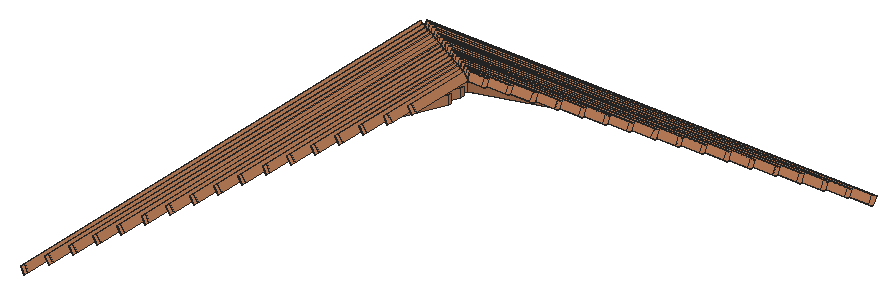
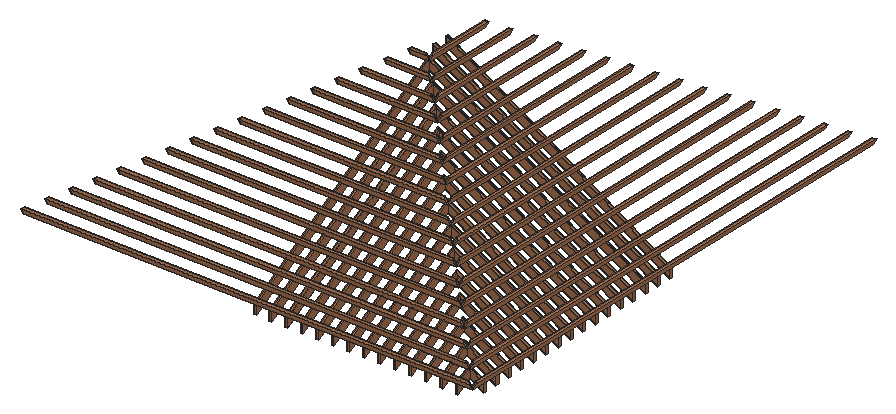
# SketchUp Ruby script. Lengths in millimetres.
U = 1.mm
M = Sketchup.active_model
def pt(a) = Geom::Point3d.new(a.map { |v| v * U })
def face(e, loops, mat)
  f = e.add_face(loops[0].map { |a| pt(a) })
  loops[1..].each { |l| e.add_face(l.map { |a| pt(a) }).erase! }
  f.material = f.back_material = mat if mat
  f
end
# faces: each face lists its corners as indices into pts; further lists are holes
def faces(e, pts, list, mat = nil) = list.each { |f| face(e, (f[0].is_a?(Array) ? f : [f]).map { |l| l.map { |i| pts[i] } }, mat) }
# xy, xz, yz: faces in a plane at the given z, y or x. An outline is a flat list of corners, or four numbers for a rectangle; further outlines are holes
def ring(l) = l.size == 4 ? [[l[0], l[1]], [l[2], l[1]], [l[2], l[3]], [l[0], l[3]]] : l.each_slice(2).to_a
def flat(e, list, mat, &to3) = list.each { |f| face(e, (f[0].is_a?(Array) ? f : [f]).map { |l| ring(l).map { |u, v| to3.(u, v) } }, mat) }
def xy(e, z, list, mat = nil) = flat(e, list, mat) { |x, y| [x, y, z] }
def xz(e, y, list, mat = nil) = flat(e, list, mat) { |x, z| [x, y, z] }
def yz(e, x, list, mat = nil) = flat(e, list, mat) { |y, z| [x, y, z] }
def lines(e, pts, list) = list.each { |a, b| e.add_line(pt(pts[a]), pt(pts[b])) }
# prism: a flat outline (further loops are holes) pulled along v
def prism(e, loops, v, mat = nil)
  f = face(e, loops, mat); d = Geom::Vector3d.new(v.map { |x| x * U })
  f.pushpull(f.normal.samedirection?(d) ? d.length : -d.length)
end
def box(e, o, s, mat = nil) = prism(e, [[o, [o[0] + s[0], o[1], o[2]], [o[0] + s[0], o[1] + s[1], o[2]], [o[0], o[1] + s[1], o[2]]]], [0, 0, s[2]], mat)
def at(x, y, z, deg = 0) = Geom::Transformation.translation(pt([x, y, z])) * Geom::Transformation.rotation(ORIGIN, Z_AXIS, deg.degrees)
def axes(o, x, y, z) = Geom::Transformation.new([*x, 0, *y, 0, *z, 0, *pt(o).to_a, 1])
def part(name) = M.definitions.add(name)
# library, detail: a bought-in or finely detailed component or shape, given as its bounding box
def library(name, o, s) = part(name).tap { |d| box(d.entities, o, s) }
def detail(e, o, s) = box(e.add_group.entities, o, s)
def put(e, d, t, mat = nil) = e.add_instance(d, t).tap { |i| i.material = mat if mat }
def group(e, t, mat = nil) = e.add_group.tap { |g| g.transformation = t; g.material = mat if mat }.entities
root = M.entities
M.materials.add("[Wood Veneer 02]").color = [190, 128, 91]
c1 = part("Group162\#1")
xy(c1.entities,0,[[-322.7,-9540.5,-381.6,-9489.5,0,-9489.5,0,-9540.5]])
xy(c1.entities,152,[[-410.5,-9540.5,-87.8,-9540.5,-87.8,-9489.5,-469.4,-9489.5]])
xz(c1.entities,-9540.5,[[-322.7,0,0,0,-87.8,152,-410.5,152]])
xz(c1.entities,-9489.5,[[-381.6,0,-469.4,152,-87.8,152,0,0]])
p = [[-381.6,-9489.5,0],[-322.7,-9540.5,0],[-410.5,-9540.5,152],[-469.4,-9489.5,152],[0,-9540.5,0],[0,-9489.5,0],
  [-87.8,-9489.5,152],[-87.8,-9540.5,152]]
faces(c1.entities,p,[[0,1,2,3],[4,5,6,7]])
c2 = part("Group115\#1")
xy(c2.entities,0,[[-381.6,-330.5,-322.7,-279.5,0,-279.5,0,-330.5]])
xy(c2.entities,152,[[-469.4,-330.5,-87.8,-330.5,-87.8,-279.5,-410.5,-279.5]])
xz(c2.entities,-330.5,[[-381.6,0,0,0,-87.8,152,-469.4,152]])
xz(c2.entities,-279.5,[[-322.7,0,-410.5,152,-87.8,152,0,0]])
p = [[-381.6,-330.5,0],[-469.4,-330.5,152],[-410.5,-279.5,152],[-322.7,-279.5,0],[-87.8,-330.5,152],[0,-330.5,0],
  [0,-279.5,0],[-87.8,-279.5,152]]
faces(c2.entities,p,[[0,1,2,3],[4,5,6,7]])
c3 = part("Group164\#1")
xy(c3.entities,0,[[-674.9,-9235.5,-733.8,-9184.5,0,-9184.5,0,-9235.5]])
xy(c3.entities,152,[[-762.7,-9235.5,-87.8,-9235.5,-87.8,-9184.5,-821.6,-9184.5]])
xz(c3.entities,-9235.5,[[-674.9,0,0,0,-87.8,152,-762.7,152]])
xz(c3.entities,-9184.5,[[-733.8,0,-821.6,152,-87.8,152,0,0]])
p = [[-674.9,-9235.5,0],[-762.7,-9235.5,152],[-821.6,-9184.5,152],[-733.8,-9184.5,0],[-87.8,-9235.5,152],[0,-9235.5,0],
  [0,-9184.5,0],[-87.8,-9184.5,152]]
faces(c3.entities,p,[[0,1,2,3],[4,5,6,7]])
c4 = part("Group166\#1")
xy(c4.entities,0,[[-1027.1,-8930.5,-1086,-8879.5,0,-8879.5,0,-8930.5]])
xy(c4.entities,152,[[-1114.9,-8930.5,-87.8,-8930.5,-87.8,-8879.5,-1173.8,-8879.5]])
xz(c4.entities,-8930.5,[[-1027.1,0,0,0,-87.8,152,-1114.9,152]])
xz(c4.entities,-8879.5,[[-1086,0,-1173.8,152,-87.8,152,0,0]])
p = [[-1086,-8879.5,0],[-1027.1,-8930.5,0],[-1114.9,-8930.5,152],[-1173.8,-8879.5,152],[0,-8930.5,0],[0,-8879.5,0],
  [-87.8,-8879.5,152],[-87.8,-8930.5,152]]
faces(c4.entities,p,[[0,1,2,3],[4,5,6,7]])
c5 = part("Group117\#1")
xy(c5.entities,0,[[-733.8,-635.5,-674.9,-584.5,0,-584.5,0,-635.5]])
xy(c5.entities,152,[[-821.6,-635.5,-87.8,-635.5,-87.8,-584.5,-762.7,-584.5]])
xz(c5.entities,-635.5,[[-733.8,0,0,0,-87.8,152,-821.6,152]])
xz(c5.entities,-584.5,[[-674.9,0,-762.7,152,-87.8,152,0,0]])
p = [[-762.7,-584.5,152],[-674.9,-584.5,0],[-733.8,-635.5,0],[-821.6,-635.5,152],[0,-584.5,0],[-87.8,-584.5,152],
  [-87.8,-635.5,152],[0,-635.5,0]]
faces(c5.entities,p,[[0,1,2,3],[4,5,6,7]])
c6 = part("Group168\#1")
xy(c6.entities,0,[[-1379.3,-8625.5,-1438.2,-8574.5,0,-8574.5,0,-8625.5]])
xy(c6.entities,152,[[-1467,-8625.5,-87.8,-8625.5,-87.8,-8574.5,-1525.9,-8574.5]])
xz(c6.entities,-8625.5,[[-1379.3,0,0,0,-87.8,152,-1467,152]])
xz(c6.entities,-8574.5,[[-1438.2,0,-1525.9,152,-87.8,152,0,0]])
p = [[-1379.3,-8625.5,0],[-1467,-8625.5,152],[-1525.9,-8574.5,152],[-1438.2,-8574.5,0],[-87.8,-8625.5,152],[0,-8625.5,0],
  [0,-8574.5,0],[-87.8,-8574.5,152]]
faces(c6.entities,p,[[0,1,2,3],[4,5,6,7]])
c7 = part("Group170\#1")
xy(c7.entities,0,[[-1731.5,-8320.5,-1790.4,-8269.5,0,-8269.5,0,-8320.5]])
xy(c7.entities,152,[[-1819.2,-8320.5,-87.8,-8320.5,-87.8,-8269.5,-1878.1,-8269.5]])
xz(c7.entities,-8320.5,[[-1731.5,0,0,0,-87.8,152,-1819.2,152]])
xz(c7.entities,-8269.5,[[-1790.4,0,-1878.1,152,-87.8,152,0,0]])
p = [[-1819.2,-8320.5,152],[-1878.1,-8269.5,152],[-1790.4,-8269.5,0],[-1731.5,-8320.5,0],[-87.8,-8269.5,152],[-87.8,-8320.5,152],
  [0,-8320.5,0],[0,-8269.5,0]]
faces(c7.entities,p,[[0,1,2,3],[4,5,6,7]])
c8 = part("Group119\#1")
xy(c8.entities,0,[[-1086,-940.5,-1027.1,-889.5,0,-889.5,0,-940.5]])
xy(c8.entities,152,[[-1173.8,-940.5,-87.8,-940.5,-87.8,-889.5,-1114.9,-889.5]])
xz(c8.entities,-940.5,[[-1086,0,0,0,-87.8,152,-1173.8,152]])
xz(c8.entities,-889.5,[[-1027.1,0,-1114.9,152,-87.8,152,0,0]])
p = [[-1114.9,-889.5,152],[-1027.1,-889.5,0],[-1086,-940.5,0],[-1173.8,-940.5,152],[0,-889.5,0],[-87.8,-889.5,152],
  [-87.8,-940.5,152],[0,-940.5,0]]
faces(c8.entities,p,[[0,1,2,3],[4,5,6,7]])
c9 = part("Group172\#1")
xy(c9.entities,0,[[-2083.7,-8015.5,-2142.5,-7964.5,0,-7964.5,0,-8015.5]])
xy(c9.entities,152,[[-2171.4,-8015.5,-87.8,-8015.5,-87.8,-7964.5,-2230.3,-7964.5]])
xz(c9.entities,-8015.5,[[-2083.7,0,0,0,-87.8,152,-2171.4,152]])
xz(c9.entities,-7964.5,[[-2142.5,0,-2230.3,152,-87.8,152,0,0]])
p = [[-2171.4,-8015.5,152],[-2230.3,-7964.5,152],[-2142.5,-7964.5,0],[-2083.7,-8015.5,0],[-87.8,-7964.5,152],[-87.8,-8015.5,152],
  [0,-8015.5,0],[0,-7964.5,0]]
faces(c9.entities,p,[[0,1,2,3],[4,5,6,7]])
c10 = part("Group174\#1")
xy(c10.entities,0,[[-2435.8,-7710.5,-2494.7,-7659.5,0,-7659.5,0,-7710.5]])
xy(c10.entities,152,[[-2523.6,-7710.5,-87.8,-7710.5,-87.8,-7659.5,-2582.5,-7659.5]])
xz(c10.entities,-7710.5,[[-2435.8,0,0,0,-87.8,152,-2523.6,152]])
xz(c10.entities,-7659.5,[[-2494.7,0,-2582.5,152,-87.8,152,0,0]])
p = [[-2435.8,-7710.5,0],[-2523.6,-7710.5,152],[-2582.5,-7659.5,152],[-2494.7,-7659.5,0],[-87.8,-7710.5,152],[0,-7710.5,0],
  [0,-7659.5,0],[-87.8,-7659.5,152]]
faces(c10.entities,p,[[0,1,2,3],[4,5,6,7]])
c11 = part("Group121\#1")
xy(c11.entities,0,[[-1438.2,-1245.5,-1379.3,-1194.5,0,-1194.5,0,-1245.5]])
xy(c11.entities,152,[[-1525.9,-1245.5,-87.8,-1245.5,-87.8,-1194.5,-1467,-1194.5]])
xz(c11.entities,-1245.5,[[-1438.2,0,0,0,-87.8,152,-1525.9,152]])
xz(c11.entities,-1194.5,[[-1379.3,0,-1467,152,-87.8,152,0,0]])
p = [[-1379.3,-1194.5,0],[-1438.2,-1245.5,0],[-1525.9,-1245.5,152],[-1467,-1194.5,152],[0,-1245.5,0],[0,-1194.5,0],
  [-87.8,-1194.5,152],[-87.8,-1245.5,152]]
faces(c11.entities,p,[[0,1,2,3],[4,5,6,7]])
c12 = part("Group176\#1")
xy(c12.entities,0,[[-2788,-7405.5,-2846.9,-7354.5,0,-7354.5,0,-7405.5]])
xy(c12.entities,152,[[-2875.8,-7405.5,-87.8,-7405.5,-87.8,-7354.5,-2934.7,-7354.5]])
xz(c12.entities,-7405.5,[[-2788,0,0,0,-87.8,152,-2875.8,152]])
xz(c12.entities,-7354.5,[[-2846.9,0,-2934.7,152,-87.8,152,0,0]])
p = [[-2788,-7405.5,0],[-2875.8,-7405.5,152],[-2934.7,-7354.5,152],[-2846.9,-7354.5,0],[-87.8,-7405.5,152],[0,-7405.5,0],
  [0,-7354.5,0],[-87.8,-7354.5,152]]
faces(c12.entities,p,[[0,1,2,3],[4,5,6,7]])
c13 = part("Group178\#1")
xy(c13.entities,0,[[-3140.2,-7100.5,-3199.1,-7049.5,0,-7049.5,0,-7100.5]])
xy(c13.entities,152,[[-3228,-7100.5,-87.8,-7100.5,-87.8,-7049.5,-3286.9,-7049.5]])
xz(c13.entities,-7100.5,[[-3140.2,0,0,0,-87.8,152,-3228,152]])
xz(c13.entities,-7049.5,[[-3199.1,0,-3286.9,152,-87.8,152,0,0]])
p = [[-3228,-7100.5,152],[-3286.9,-7049.5,152],[-3199.1,-7049.5,0],[-3140.2,-7100.5,0],[-87.8,-7049.5,152],[-87.8,-7100.5,152],
  [0,-7100.5,0],[0,-7049.5,0]]
faces(c13.entities,p,[[0,1,2,3],[4,5,6,7]])
c14 = part("Group123\#1")
xy(c14.entities,0,[[-1790.4,-1550.5,-1731.5,-1499.5,0,-1499.5,0,-1550.5]])
xy(c14.entities,152,[[-1878.1,-1550.5,-87.8,-1550.5,-87.8,-1499.5,-1819.2,-1499.5]])
xz(c14.entities,-1550.5,[[-1790.4,0,0,0,-87.8,152,-1878.1,152]])
xz(c14.entities,-1499.5,[[-1731.5,0,-1819.2,152,-87.8,152,0,0]])
p = [[-1878.1,-1550.5,152],[-1819.2,-1499.5,152],[-1731.5,-1499.5,0],[-1790.4,-1550.5,0],[-87.8,-1499.5,152],[-87.8,-1550.5,152],
  [0,-1550.5,0],[0,-1499.5,0]]
faces(c14.entities,p,[[0,1,2,3],[4,5,6,7]])
c15 = part("Group180\#1")
xy(c15.entities,0,[[-3492.4,-6795.5,-3551.3,-6744.5,0,-6744.5,0,-6795.5]])
xy(c15.entities,152,[[-3580.1,-6795.5,-87.8,-6795.5,-87.8,-6744.5,-3639,-6744.5]])
xz(c15.entities,-6795.5,[[-3492.4,0,0,0,-87.8,152,-3580.1,152]])
xz(c15.entities,-6744.5,[[-3551.3,0,-3639,152,-87.8,152,0,0]])
p = [[-3551.3,-6744.5,0],[-3492.4,-6795.5,0],[-3580.1,-6795.5,152],[-3639,-6744.5,152],[0,-6795.5,0],[0,-6744.5,0],
  [-87.8,-6744.5,152],[-87.8,-6795.5,152]]
faces(c15.entities,p,[[0,1,2,3],[4,5,6,7]])
c16 = part("Group182\#1")
xy(c16.entities,0,[[-3844.6,-6490.5,-3903.5,-6439.5,0,-6439.5,0,-6490.5]])
xy(c16.entities,152,[[-3932.3,-6490.5,-87.8,-6490.5,-87.8,-6439.5,-3991.2,-6439.5]])
xz(c16.entities,-6490.5,[[-3844.6,0,0,0,-87.8,152,-3932.3,152]])
xz(c16.entities,-6439.5,[[-3903.5,0,-3991.2,152,-87.8,152,0,0]])
p = [[-3903.5,-6439.5,0],[-3844.6,-6490.5,0],[-3932.3,-6490.5,152],[-3991.2,-6439.5,152],[0,-6490.5,0],[0,-6439.5,0],
  [-87.8,-6439.5,152],[-87.8,-6490.5,152]]
faces(c16.entities,p,[[0,1,2,3],[4,5,6,7]])
c17 = part("Group125\#1")
xy(c17.entities,0,[[-2142.5,-1855.5,-2083.7,-1804.5,0,-1804.5,0,-1855.5]])
xy(c17.entities,152,[[-2230.3,-1855.5,-87.8,-1855.5,-87.8,-1804.5,-2171.4,-1804.5]])
xz(c17.entities,-1855.5,[[-2142.5,0,0,0,-87.8,152,-2230.3,152]])
xz(c17.entities,-1804.5,[[-2083.7,0,-2171.4,152,-87.8,152,0,0]])
p = [[-2171.4,-1804.5,152],[-2083.7,-1804.5,0],[-2142.5,-1855.5,0],[-2230.3,-1855.5,152],[0,-1804.5,0],[-87.8,-1804.5,152],
  [-87.8,-1855.5,152],[0,-1855.5,0]]
faces(c17.entities,p,[[0,1,2,3],[4,5,6,7]])
c18 = part("Group184\#1")
xy(c18.entities,0,[[-4196.8,-6185.5,-4255.6,-6134.5,0,-6134.5,0,-6185.5]])
xy(c18.entities,152,[[-4284.5,-6185.5,-87.8,-6185.5,-87.8,-6134.5,-4343.4,-6134.5]])
xz(c18.entities,-6185.5,[[-4196.8,0,0,0,-87.8,152,-4284.5,152]])
xz(c18.entities,-6134.5,[[-4255.6,0,-4343.4,152,-87.8,152,0,0]])
p = [[-4343.4,-6134.5,152],[-4255.6,-6134.5,0],[-4196.8,-6185.5,0],[-4284.5,-6185.5,152],[0,-6134.5,0],[-87.8,-6134.5,152],
  [-87.8,-6185.5,152],[0,-6185.5,0]]
faces(c18.entities,p,[[0,1,2,3],[4,5,6,7]])
c19 = part("Group186\#1")
xy(c19.entities,0,[[-4548.9,-5880.5,-4607.8,-5829.5,0,-5829.5,0,-5880.5]])
xy(c19.entities,152,[[-4636.7,-5880.5,-87.8,-5880.5,-87.8,-5829.5,-4695.6,-5829.5]])
xz(c19.entities,-5880.5,[[-4548.9,0,0,0,-87.8,152,-4636.7,152]])
xz(c19.entities,-5829.5,[[-4607.8,0,-4695.6,152,-87.8,152,0,0]])
p = [[-4607.8,-5829.5,0],[-4548.9,-5880.5,0],[-4636.7,-5880.5,152],[-4695.6,-5829.5,152],[0,-5880.5,0],[0,-5829.5,0],
  [-87.8,-5829.5,152],[-87.8,-5880.5,152]]
faces(c19.entities,p,[[0,1,2,3],[4,5,6,7]])
c20 = part("Group195\#1")
prism(c20.entities,[[[-4865.8,-2495.1,0],[4865.8,-2495.1,0],[4910,-2546.1,0],[-4910,-2546.1,0]]],[0,0,152])
c21 = part("Group196\#1")
prism(c21.entities,[[[4645.9,-2241.1,0],[-4645.9,-2241.1,0],[-4601.7,-2190.1,0],[4601.7,-2190.1,0]]],[0,0,152])
c22 = part("Group197\#1")
prism(c22.entities,[[[-4337.6,-1885.1,0],[4337.6,-1885.1,0],[4381.7,-1936.1,0],[-4381.7,-1936.1,0]]],[0,0,152])
c23 = part("Group198\#1")
prism(c23.entities,[[[-4073.4,-1580.1,0],[4073.4,-1580.1,0],[4117.6,-1631.1,0],[-4117.6,-1631.1,0]]],[0,0,152])
c24 = part("Group199\#1")
prism(c24.entities,[[[-3809.3,-1275.1,0],[3809.3,-1275.1,0],[3853.4,-1326.1,0],[-3853.4,-1326.1,0]]],[0,0,152])
c25 = part("Group200\#1")
prism(c25.entities,[[[3589.3,-1021.1,0],[-3589.3,-1021.1,0],[-3545.1,-970.1,0],[3545.1,-970.1,0]]],[0,0,152])
c26 = part("Group201\#1")
prism(c26.entities,[[[3325.2,-716.1,0],[-3325.2,-716.1,0],[-3281,-665.1,0],[3281,-665.1,0]]],[0,0,152])
c27 = part("Group202\#1")
prism(c27.entities,[[[-3016.9,-360.1,0],[3016.9,-360.1,0],[3061,-411.1,0],[-3061,-411.1,0]]],[0,0,152])
c28 = part("Group203\#1")
prism(c28.entities,[[[2796.9,-106.1,0],[-2796.9,-106.1,0],[-2752.7,-55.1,0],[2752.7,-55.1,0]]],[0,0,152])
c29 = part("Group204\#1")
prism(c29.entities,[[[2532.8,198.9,0],[-2532.8,198.9,0],[-2488.6,249.9,0],[2488.6,249.9,0]]],[0,0,152])
c30 = part("Group205\#1")
prism(c30.entities,[[[-2224.5,554.9,0],[2224.5,554.9,0],[2268.6,503.9,0],[-2268.6,503.9,0]]],[0,0,152])
c31 = part("Group206\#1")
prism(c31.entities,[[[-1960.3,859.9,0],[1960.3,859.9,0],[2004.5,808.9,0],[-2004.5,808.9,0]]],[0,0,152])
c32 = part("Group207\#1")
prism(c32.entities,[[[-1696.2,1164.9,0],[1696.2,1164.9,0],[1740.3,1113.9,0],[-1740.3,1113.9,0]]],[0,0,152])
c33 = part("Group208\#1")
prism(c33.entities,[[[-1432,1469.9,0],[1432,1469.9,0],[1476.2,1418.9,0],[-1476.2,1418.9,0]]],[0,0,152])
c34 = part("Group209\#1")
prism(c34.entities,[[[-1167.9,1774.9,0],[1167.9,1774.9,0],[1212.1,1723.9,0],[-1212.1,1723.9,0]]],[0,0,152])
c35 = part("Group210\#1")
prism(c35.entities,[[[-903.8,2079.9,0],[903.8,2079.9,0],[947.9,2028.9,0],[-947.9,2028.9,0]]],[0,0,152])
c36 = part("Group211\#1")
prism(c36.entities,[[[-639.6,2384.9,0],[639.6,2384.9,0],[683.8,2333.9,0],[-683.8,2333.9,0]]],[0,0,152])
c37 = part("Group193\#2")
put(c37.entities,c20,at(0,0,0))
put(c37.entities,c21,at(0,0,0))
put(c37.entities,c22,at(0,0,0))
put(c37.entities,c23,at(0,0,0))
put(c37.entities,c24,at(0,0,0))
put(c37.entities,c25,at(0,0,0))
put(c37.entities,c26,at(0,0,0))
put(c37.entities,c27,at(0,0,0))
put(c37.entities,c28,at(0,0,0))
put(c37.entities,c29,at(0,0,0))
put(c37.entities,c30,at(0,0,0))
put(c37.entities,c31,at(0,0,0))
put(c37.entities,c32,at(0,0,0))
put(c37.entities,c33,at(0,0,0))
put(c37.entities,c34,at(0,0,0))
put(c37.entities,c35,at(0,0,0))
put(c37.entities,c36,at(0,0,0))
c38 = part("Group127\#1")
xy(c38.entities,0,[[-2494.7,-2160.5,-2435.8,-2109.5,0,-2109.5,0,-2160.5]])
xy(c38.entities,152,[[-2582.5,-2160.5,-87.8,-2160.5,-87.8,-2109.5,-2523.6,-2109.5]])
xz(c38.entities,-2160.5,[[-2494.7,0,0,0,-87.8,152,-2582.5,152]])
xz(c38.entities,-2109.5,[[-2435.8,0,-2523.6,152,-87.8,152,0,0]])
p = [[-2435.8,-2109.5,0],[-2494.7,-2160.5,0],[-2582.5,-2160.5,152],[-2523.6,-2109.5,152],[0,-2160.5,0],[0,-2109.5,0],
  [-87.8,-2109.5,152],[-87.8,-2160.5,152]]
faces(c38.entities,p,[[0,1,2,3],[4,5,6,7]])
c39 = part("Group188\#1")
xy(c39.entities,0,[[-4901.1,-5575.5,-4960,-5524.5,0,-5524.5,0,-5575.5]])
xy(c39.entities,152,[[-4988.9,-5575.5,-87.8,-5575.5,-87.8,-5524.5,-5047.8,-5524.5]])
xz(c39.entities,-5575.5,[[-4901.1,0,0,0,-87.8,152,-4988.9,152]])
xz(c39.entities,-5524.5,[[-4960,0,-5047.8,152,-87.8,152,0,0]])
p = [[-4960,-5524.5,0],[-4901.1,-5575.5,0],[-4988.9,-5575.5,152],[-5047.8,-5524.5,152],[0,-5575.5,0],[0,-5524.5,0],
  [-87.8,-5524.5,152],[-87.8,-5575.5,152]]
faces(c39.entities,p,[[0,1,2,3],[4,5,6,7]])
c40 = part("Group192\#1")
prism(c40.entities,[[[-87.8,-4965.5,152],[-5180,-4965.5,152],[-5092.2,-4965.5,0],[0,-4965.5,0]]],[0,51,0])
c41 = part("Group190\#1")
prism(c41.entities,[[[-5180,-5219.5,152],[-87.8,-5219.5,152],[0,-5219.5,0],[-5092.2,-5219.5,0]]],[0,-51,0])
c42 = part("Group129\#1")
xy(c42.entities,0,[[-2846.9,-2465.5,-2788,-2414.5,0,-2414.5,0,-2465.5]])
xy(c42.entities,152,[[-2934.7,-2465.5,-87.8,-2465.5,-87.8,-2414.5,-2875.8,-2414.5]])
xz(c42.entities,-2465.5,[[-2846.9,0,0,0,-87.8,152,-2934.7,152]])
xz(c42.entities,-2414.5,[[-2788,0,-2875.8,152,-87.8,152,0,0]])
p = [[-2934.7,-2465.5,152],[-2875.8,-2414.5,152],[-2788,-2414.5,0],[-2846.9,-2465.5,0],[-87.8,-2414.5,152],[-87.8,-2465.5,152],
  [0,-2465.5,0],[0,-2414.5,0]]
faces(c42.entities,p,[[0,1,2,3],[4,5,6,7]])
c43 = part("Group131\#1")
xy(c43.entities,0,[[-3199.1,-2770.5,-3140.2,-2719.5,0,-2719.5,0,-2770.5]])
xy(c43.entities,152,[[-3286.9,-2770.5,-87.8,-2770.5,-87.8,-2719.5,-3228,-2719.5]])
xz(c43.entities,-2770.5,[[-3199.1,0,0,0,-87.8,152,-3286.9,152]])
xz(c43.entities,-2719.5,[[-3140.2,0,-3228,152,-87.8,152,0,0]])
p = [[-3140.2,-2719.5,0],[-3199.1,-2770.5,0],[-3286.9,-2770.5,152],[-3228,-2719.5,152],[0,-2770.5,0],[0,-2719.5,0],
  [-87.8,-2719.5,152],[-87.8,-2770.5,152]]
faces(c43.entities,p,[[0,1,2,3],[4,5,6,7]])
c44 = part("Group133\#1")
xy(c44.entities,0,[[-3551.3,-3075.5,-3492.4,-3024.5,0,-3024.5,0,-3075.5]])
xy(c44.entities,152,[[-3639,-3075.5,-87.8,-3075.5,-87.8,-3024.5,-3580.1,-3024.5]])
xz(c44.entities,-3075.5,[[-3551.3,0,0,0,-87.8,152,-3639,152]])
xz(c44.entities,-3024.5,[[-3492.4,0,-3580.1,152,-87.8,152,0,0]])
p = [[-3551.3,-3075.5,0],[-3639,-3075.5,152],[-3580.1,-3024.5,152],[-3492.4,-3024.5,0],[-87.8,-3075.5,152],[0,-3075.5,0],
  [0,-3024.5,0],[-87.8,-3024.5,152]]
faces(c44.entities,p,[[0,1,2,3],[4,5,6,7]])
c45 = part("Group135\#1")
xy(c45.entities,0,[[-3903.5,-3380.5,-3844.6,-3329.5,0,-3329.5,0,-3380.5]])
xy(c45.entities,152,[[-3991.2,-3380.5,-87.8,-3380.5,-87.8,-3329.5,-3932.3,-3329.5]])
xz(c45.entities,-3380.5,[[-3903.5,0,0,0,-87.8,152,-3991.2,152]])
xz(c45.entities,-3329.5,[[-3844.6,0,-3932.3,152,-87.8,152,0,0]])
p = [[-3903.5,-3380.5,0],[-3991.2,-3380.5,152],[-3932.3,-3329.5,152],[-3844.6,-3329.5,0],[-87.8,-3380.5,152],[0,-3380.5,0],
  [0,-3329.5,0],[-87.8,-3329.5,152]]
faces(c45.entities,p,[[0,1,2,3],[4,5,6,7]])
c46 = part("Group137\#1")
xy(c46.entities,0,[[-4255.6,-3685.5,-4196.8,-3634.5,0,-3634.5,0,-3685.5]])
xy(c46.entities,152,[[-4343.4,-3685.5,-87.8,-3685.5,-87.8,-3634.5,-4284.5,-3634.5]])
xz(c46.entities,-3685.5,[[-4255.6,0,0,0,-87.8,152,-4343.4,152]])
xz(c46.entities,-3634.5,[[-4196.8,0,-4284.5,152,-87.8,152,0,0]])
p = [[-4343.4,-3685.5,152],[-4284.5,-3634.5,152],[-4196.8,-3634.5,0],[-4255.6,-3685.5,0],[-87.8,-3634.5,152],[-87.8,-3685.5,152],
  [0,-3685.5,0],[0,-3634.5,0]]
faces(c46.entities,p,[[0,1,2,3],[4,5,6,7]])
c47 = part("Group139\#1")
xy(c47.entities,0,[[-4607.8,-3990.5,-4548.9,-3939.5,0,-3939.5,0,-3990.5]])
xy(c47.entities,152,[[-4695.6,-3990.5,-87.8,-3990.5,-87.8,-3939.5,-4636.7,-3939.5]])
xz(c47.entities,-3990.5,[[-4607.8,0,0,0,-87.8,152,-4695.6,152]])
xz(c47.entities,-3939.5,[[-4548.9,0,-4636.7,152,-87.8,152,0,0]])
p = [[-4695.6,-3990.5,152],[-4636.7,-3939.5,152],[-4548.9,-3939.5,0],[-4607.8,-3990.5,0],[-87.8,-3939.5,152],[-87.8,-3990.5,152],
  [0,-3990.5,0],[0,-3939.5,0]]
faces(c47.entities,p,[[0,1,2,3],[4,5,6,7]])
c48 = part("Group141\#1")
xy(c48.entities,0,[[-4960,-4295.5,-4901.1,-4244.5,0,-4244.5,0,-4295.5]])
xy(c48.entities,152,[[-5047.8,-4295.5,-87.8,-4295.5,-87.8,-4244.5,-4988.9,-4244.5]])
xz(c48.entities,-4295.5,[[-4960,0,0,0,-87.8,152,-5047.8,152]])
xz(c48.entities,-4244.5,[[-4901.1,0,-4988.9,152,-87.8,152,0,0]])
p = [[-5047.8,-4295.5,152],[-4988.9,-4244.5,152],[-4901.1,-4244.5,0],[-4960,-4295.5,0],[-87.8,-4244.5,152],[-87.8,-4295.5,152],
  [0,-4295.5,0],[0,-4244.5,0]]
faces(c48.entities,p,[[0,1,2,3],[4,5,6,7]])
c49 = part("Group143\#1")
prism(c49.entities,[[[-4365.8,-2495.1,0],[4365.8,-2495.1,0],[4410,-2546.1,0],[-4410,-2546.1,0]]],[0,0,152])
c50 = part("Group144\#1")
prism(c50.entities,[[[4145.9,-2241.1,0],[-4145.9,-2241.1,0],[-4101.7,-2190.1,0],[4101.7,-2190.1,0]]],[0,0,152])
c51 = part("Group145\#1")
prism(c51.entities,[[[3881.7,-1936.1,0],[-3881.7,-1936.1,0],[-3837.6,-1885.1,0],[3837.6,-1885.1,0]]],[0,0,152])
c52 = part("Group146\#1")
prism(c52.entities,[[[3617.6,-1631.1,0],[-3617.6,-1631.1,0],[-3573.4,-1580.1,0],[3573.4,-1580.1,0]]],[0,0,152])
c53 = part("Group147\#1")
prism(c53.entities,[[[3353.4,-1326.1,0],[-3353.4,-1326.1,0],[-3309.3,-1275.1,0],[3309.3,-1275.1,0]]],[0,0,152])
c54 = part("Group148\#1")
prism(c54.entities,[[[3089.3,-1021.1,0],[-3089.3,-1021.1,0],[-3045.1,-970.1,0],[3045.1,-970.1,0]]],[0,0,152])
c55 = part("Group149\#1")
prism(c55.entities,[[[2825.2,-716.1,0],[-2825.2,-716.1,0],[-2781,-665.1,0],[2781,-665.1,0]]],[0,0,152])
c56 = part("Group150\#1")
prism(c56.entities,[[[2561,-411.1,0],[-2561,-411.1,0],[-2516.9,-360.1,0],[2516.9,-360.1,0]]],[0,0,152])
c57 = part("Group151\#1")
prism(c57.entities,[[[-2252.7,-55.1,0],[2252.7,-55.1,0],[2296.9,-106.1,0],[-2296.9,-106.1,0]]],[0,0,152])
c58 = part("Group152\#1")
prism(c58.entities,[[[-1988.6,249.9,0],[1988.6,249.9,0],[2032.8,198.9,0],[-2032.8,198.9,0]]],[0,0,152])
c59 = part("Group153\#1")
prism(c59.entities,[[[1768.6,503.9,0],[-1768.6,503.9,0],[-1724.5,554.9,0],[1724.5,554.9,0]]],[0,0,152])
c60 = part("Group154\#1")
prism(c60.entities,[[[1504.5,808.9,0],[-1504.5,808.9,0],[-1460.3,859.9,0],[1460.3,859.9,0]]],[0,0,152])
c61 = part("Group155\#1")
prism(c61.entities,[[[-1196.2,1164.9,0],[1196.2,1164.9,0],[1240.3,1113.9,0],[-1240.3,1113.9,0]]],[0,0,152])
c62 = part("Group156\#1")
prism(c62.entities,[[[-932,1469.9,0],[932,1469.9,0],[976.2,1418.9,0],[-976.2,1418.9,0]]],[0,0,152])
c63 = part("Group157\#1")
prism(c63.entities,[[[-667.9,1774.9,0],[667.9,1774.9,0],[712.1,1723.9,0],[-712.1,1723.9,0]]],[0,0,152])
c64 = part("Group158\#1")
prism(c64.entities,[[[447.9,2028.9,0],[-447.9,2028.9,0],[-403.8,2079.9,0],[403.8,2079.9,0]]],[0,0,152])
c65 = part("Group159\#1")
prism(c65.entities,[[[183.8,2333.9,0],[-183.8,2333.9,0],[-139.6,2384.9,0],[139.6,2384.9,0]]],[0,0,152])
c66 = part("Group141\#2")
put(c66.entities,c49,at(0,0,0))
put(c66.entities,c50,at(0,0,0))
put(c66.entities,c51,at(0,0,0))
put(c66.entities,c52,at(0,0,0))
put(c66.entities,c53,at(0,0,0))
put(c66.entities,c54,at(0,0,0))
put(c66.entities,c55,at(0,0,0))
put(c66.entities,c56,at(0,0,0))
put(c66.entities,c57,at(0,0,0))
put(c66.entities,c58,at(0,0,0))
put(c66.entities,c59,at(0,0,0))
put(c66.entities,c60,at(0,0,0))
put(c66.entities,c61,at(0,0,0))
put(c66.entities,c62,at(0,0,0))
put(c66.entities,c63,at(0,0,0))
put(c66.entities,c64,at(0,0,0))
put(c66.entities,c65,at(0,0,0))
put(root,c1,axes([1303.3,1287,3149.6],[-0.86603,0,-0.5],[0,-1,0],[-0.5,0,0.86603]),"[Wood Veneer 02]")
put(root,c2,axes([1303.3,11107,3149.6],[0,0.86603,-0.5],[-1,0,0],[0,0.5,0.86603]),"[Wood Veneer 02]")
put(root,c3,axes([1303.3,1287,3149.6],[-0.86603,0,-0.5],[0,-1,0],[-0.5,0,0.86603]),"[Wood Veneer 02]")
put(root,c4,axes([1303.3,1287,3149.6],[-0.86603,0,-0.5],[0,-1,0],[-0.5,0,0.86603]),"[Wood Veneer 02]")
put(root,c5,axes([1303.3,11107,3149.6],[0,0.86603,-0.5],[-1,0,0],[0,0.5,0.86603]),"[Wood Veneer 02]")
put(root,c6,axes([1303.3,1287,3149.6],[-0.86603,0,-0.5],[0,-1,0],[-0.5,0,0.86603]),"[Wood Veneer 02]")
put(root,c7,axes([1303.3,1287,3149.6],[-0.86603,0,-0.5],[0,-1,0],[-0.5,0,0.86603]),"[Wood Veneer 02]")
put(root,c8,axes([1303.3,11107,3149.6],[0,0.86603,-0.5],[-1,0,0],[0,0.5,0.86603]),"[Wood Veneer 02]")
put(root,c9,axes([1303.3,1287,3149.6],[-0.86603,0,-0.5],[0,-1,0],[-0.5,0,0.86603]),"[Wood Veneer 02]")
put(root,c10,axes([1303.3,1287,3149.6],[-0.86603,0,-0.5],[0,-1,0],[-0.5,0,0.86603]),"[Wood Veneer 02]")
put(root,c11,axes([1303.3,11107,3149.6],[0,0.86603,-0.5],[-1,0,0],[0,0.5,0.86603]),"[Wood Veneer 02]")
put(root,c12,axes([1303.3,1287,3149.6],[-0.86603,0,-0.5],[0,-1,0],[-0.5,0,0.86603]),"[Wood Veneer 02]")
put(root,c13,axes([1303.3,1287,3149.6],[-0.86603,0,-0.5],[0,-1,0],[-0.5,0,0.86603]),"[Wood Veneer 02]")
put(root,c14,axes([1303.3,11107,3149.6],[0,0.86603,-0.5],[-1,0,0],[0,0.5,0.86603]),"[Wood Veneer 02]")
put(root,c15,axes([1303.3,1287,3149.6],[-0.86603,0,-0.5],[0,-1,0],[-0.5,0,0.86603]),"[Wood Veneer 02]")
put(root,c16,axes([1303.3,1287,3149.6],[-0.86603,0,-0.5],[0,-1,0],[-0.5,0,0.86603]),"[Wood Veneer 02]")
put(root,c17,axes([1303.3,11107,3149.6],[0,0.86603,-0.5],[-1,0,0],[0,0.5,0.86603]),"[Wood Veneer 02]")
put(root,c18,axes([1303.3,1287,3149.6],[-0.86603,0,-0.5],[0,-1,0],[-0.5,0,0.86603]),"[Wood Veneer 02]")
put(root,c19,axes([1303.3,1287,3149.6],[-0.86603,0,-0.5],[0,-1,0],[-0.5,0,0.86603]),"[Wood Veneer 02]")
put(root,c37,axes([3508.3,6197,4598.2],[0,-1,0],[0.86603,0,0.5],[-0.5,0,0.86603]),"[Wood Veneer 02]")
put(root,c38,axes([1303.3,11107,3149.6],[0,0.86603,-0.5],[-1,0,0],[0,0.5,0.86603]),"[Wood Veneer 02]")
put(root,c39,axes([1303.3,1287,3149.6],[-0.86603,0,-0.5],[0,-1,0],[-0.5,0,0.86603]),"[Wood Veneer 02]")
put(root,c40,axes([1303.3,1287,3149.6],[-0.86603,0,-0.5],[0,-1,0],[-0.5,0,0.86603]),"[Wood Veneer 02]")
put(root,c41,axes([1303.3,1287,3149.6],[-0.86603,0,-0.5],[0,-1,0],[-0.5,0,0.86603]),"[Wood Veneer 02]")
put(root,c42,axes([1303.3,11107,3149.6],[0,0.86603,-0.5],[-1,0,0],[0,0.5,0.86603]),"[Wood Veneer 02]")
put(root,c43,axes([1303.3,11107,3149.6],[0,0.86603,-0.5],[-1,0,0],[0,0.5,0.86603]),"[Wood Veneer 02]")
put(root,c44,axes([1303.3,11107,3149.6],[0,0.86603,-0.5],[-1,0,0],[0,0.5,0.86603]),"[Wood Veneer 02]")
put(root,c45,axes([1303.3,11107,3149.6],[0,0.86603,-0.5],[-1,0,0],[0,0.5,0.86603]),"[Wood Veneer 02]")
put(root,c46,axes([1303.3,11107,3149.6],[0,0.86603,-0.5],[-1,0,0],[0,0.5,0.86603]),"[Wood Veneer 02]")
put(root,c47,axes([1303.3,11107,3149.6],[0,0.86603,-0.5],[-1,0,0],[0,0.5,0.86603]),"[Wood Veneer 02]")
put(root,c48,axes([1303.3,11107,3149.6],[0,0.86603,-0.5],[-1,0,0],[0,0.5,0.86603]),"[Wood Veneer 02]")
put(root,c66,axes([5713.3,8902,4598.2],[-1,0,0],[0,-0.86603,0.5],[0,0.5,0.86603]),"[Wood Veneer 02]")
